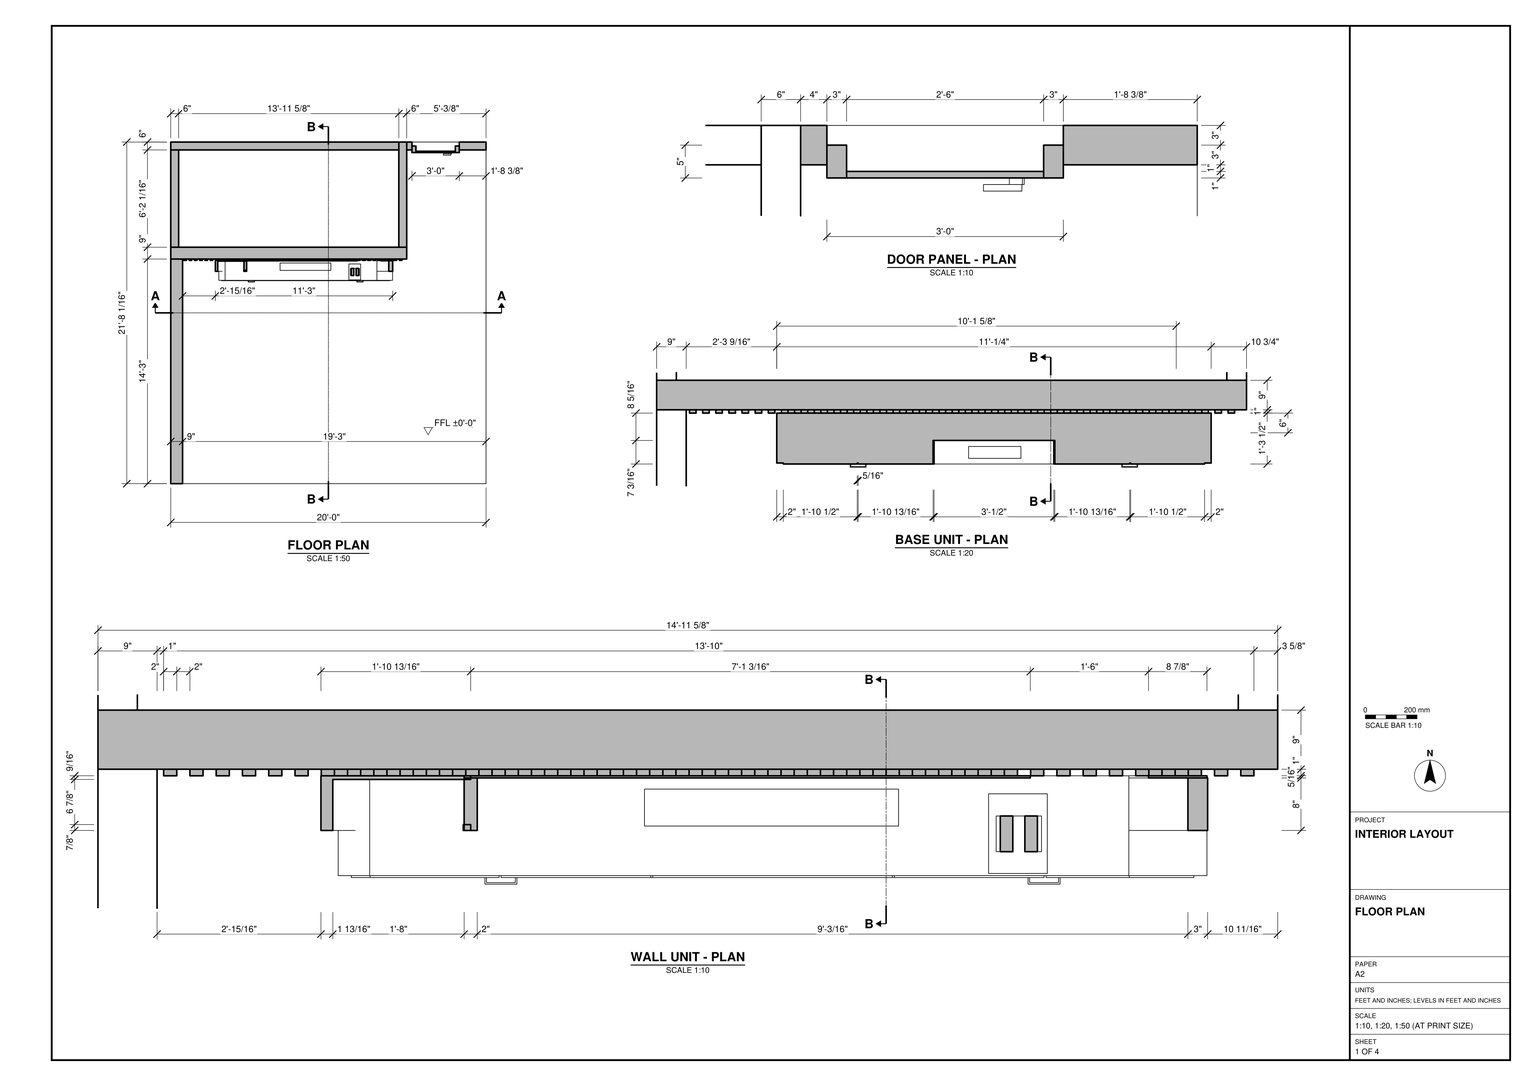
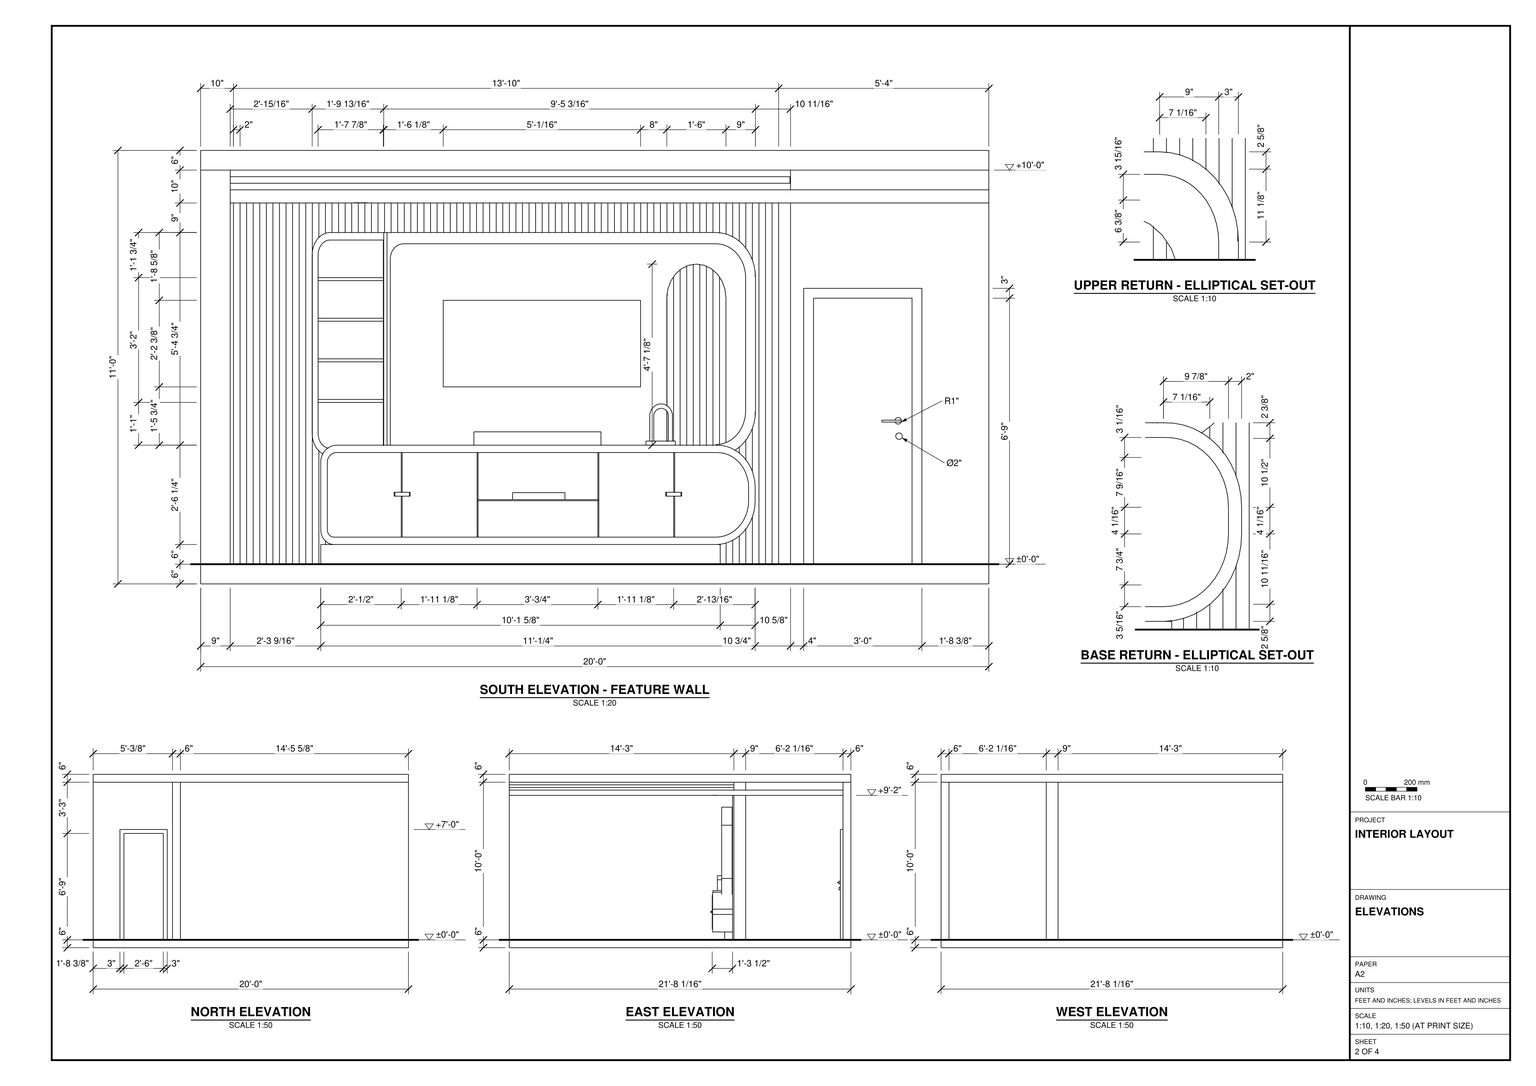
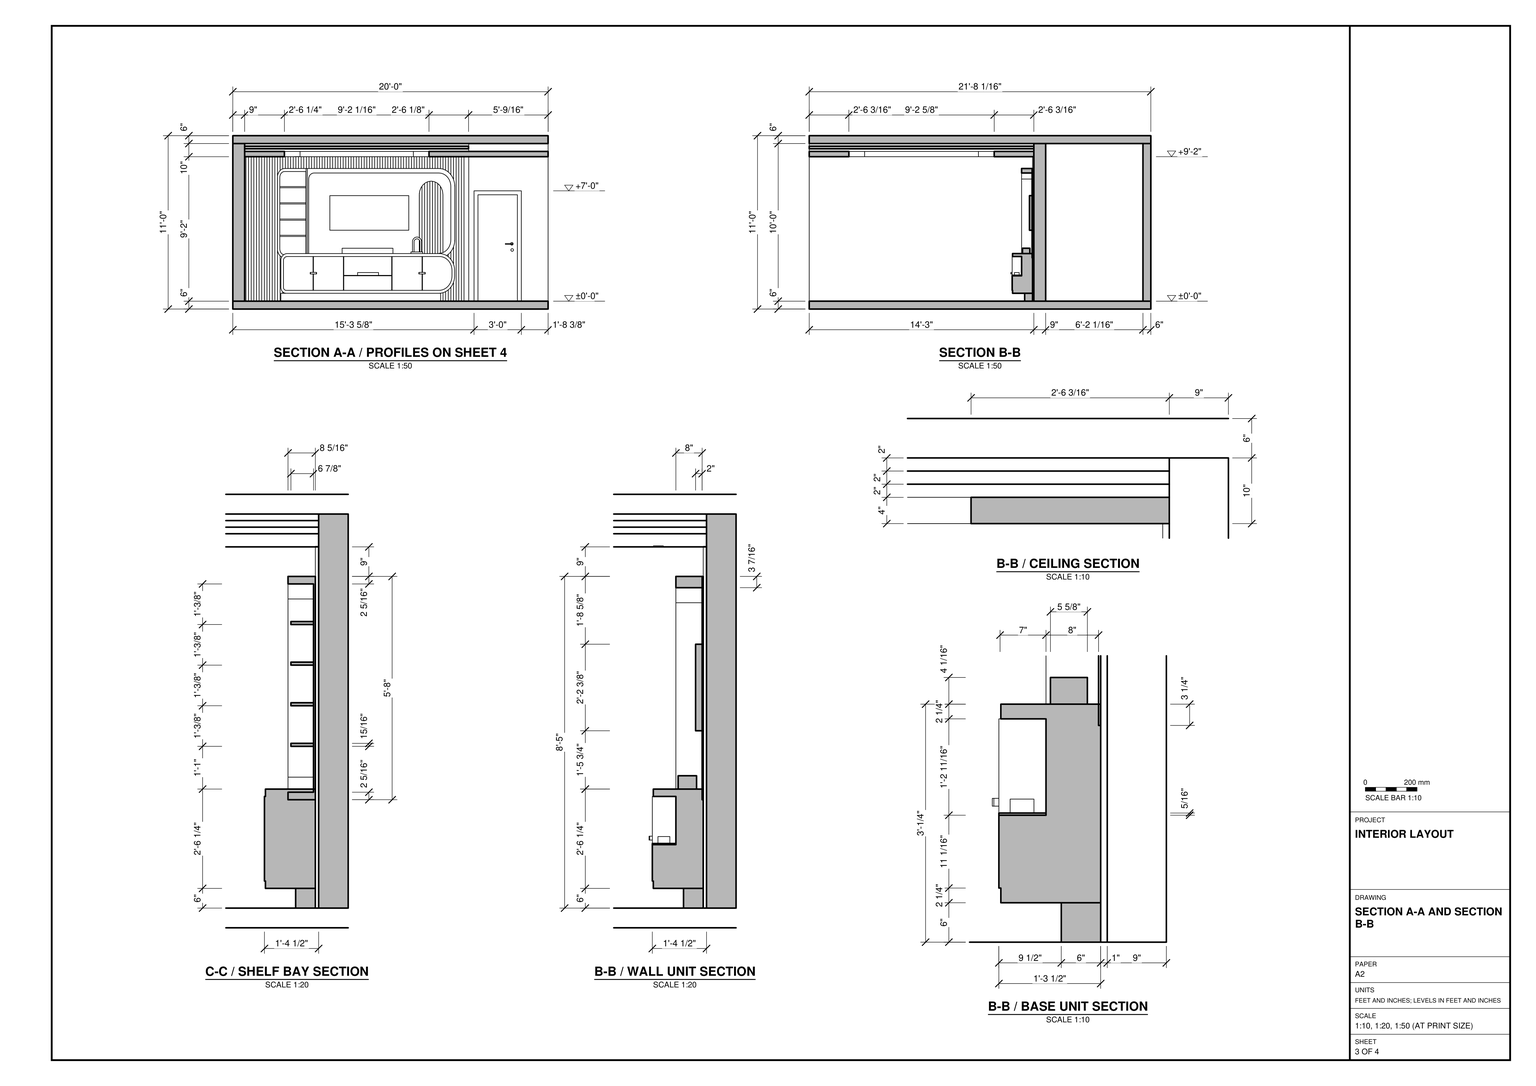
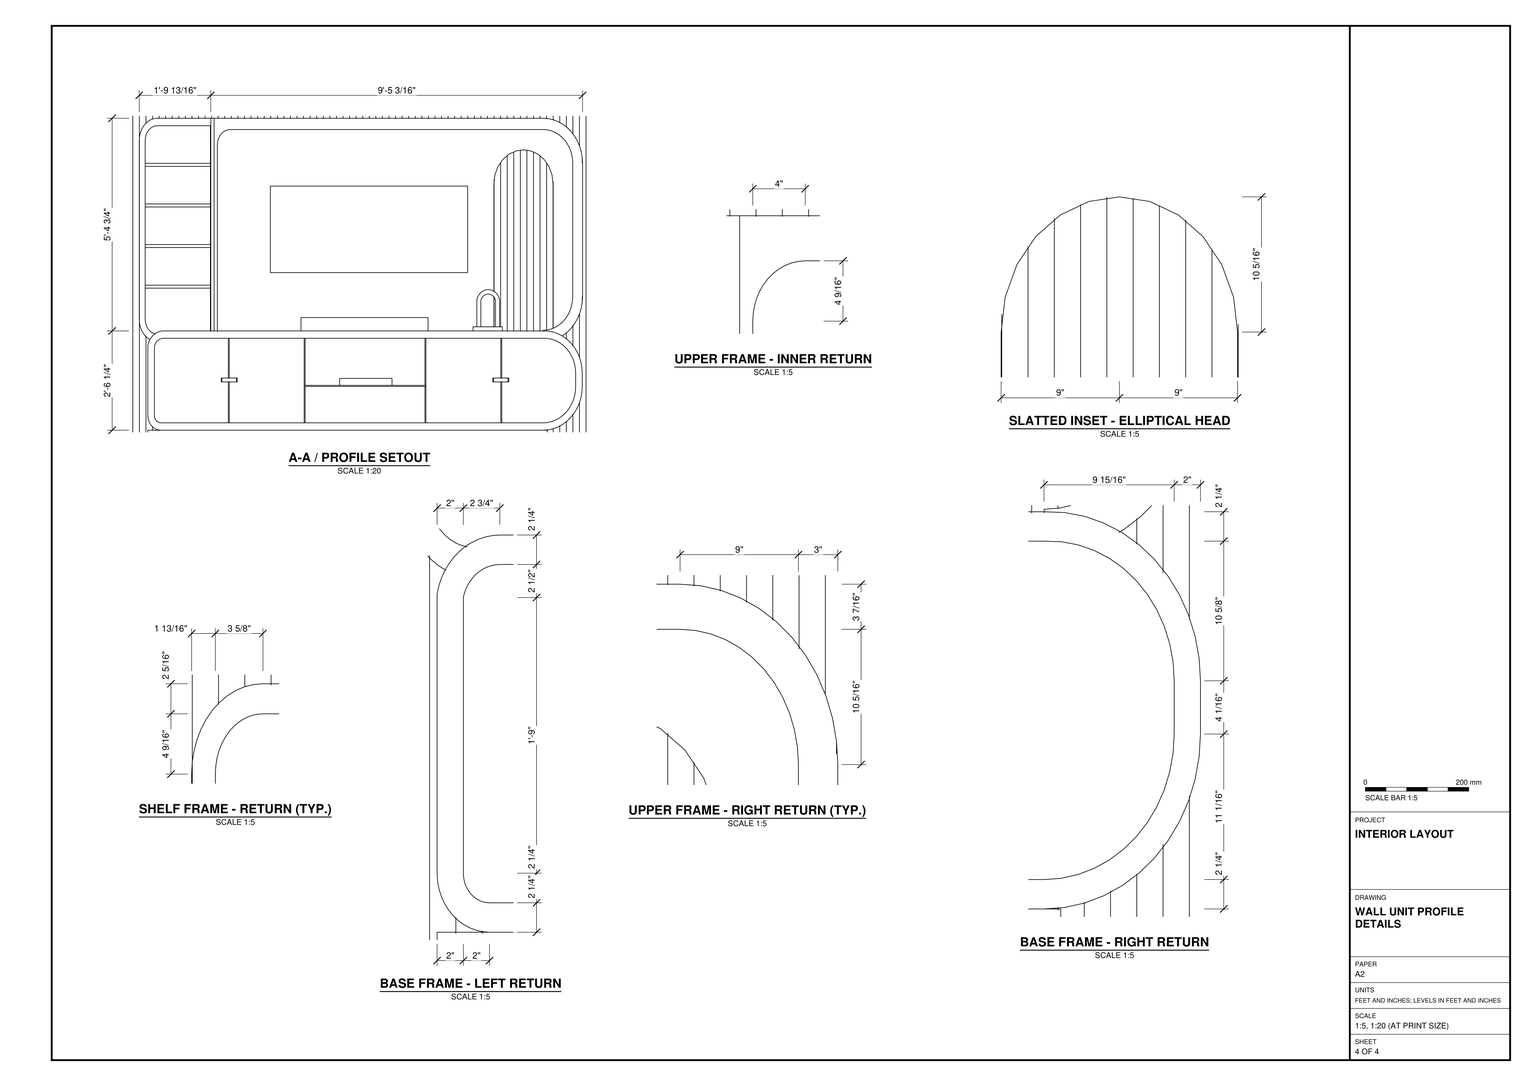
Build the single-storey interior in SketchUp using task_files/diagram_01.pdf. Work in feet and inches. The overall model is 20'-0" wide, 21'-8 1/16" deep and 11'-0" high, with the finished floor at ±0'-0".

Lay out the front room and the shallower space behind the transverse feature wall. Follow the plan for the 9" and 6" wall thicknesses, wall returns and framed door to the right of the joinery. Model the floor and upper slabs and the stepped ceiling below the upper slab, using the sections to set their heights.

Use the south elevation to lay out the vertical slats, low cabinet and upper wall unit. Set the cabinet on its recessed support and model its divided fronts, central recess and rounded right end. Above it, form the narrow open shelf bay on the left, the screen panel in the middle and the arched slatted inset on the right. Use the enlarged plans and sections for the joinery depths and the elliptical details for the curved returns. Decor and loose items may be any suitable library components.

Keep walls, slabs, ceiling and individual furniture or joinery pieces in separate groups or components, and use components for repeated parts. Save one SketchUp model as output_files/interior_with_a_curved_media_wall_and_fitted_cabinetry.skp.

# SketchUp Ruby script. Lengths in inches.
U = 1.inch
M = Sketchup.active_model
def pt(a) = Geom::Point3d.new(a.map { |v| v * U })
def face(e, loops, mat)
  f = e.add_face(loops[0].map { |a| pt(a) })
  loops[1..].each { |l| e.add_face(l.map { |a| pt(a) }).erase! }
  f.material = f.back_material = mat if mat
  f
end
# faces: each face lists its corners as indices into pts; further lists are holes
def faces(e, pts, list, mat = nil) = list.each { |f| face(e, (f[0].is_a?(Array) ? f : [f]).map { |l| l.map { |i| pts[i] } }, mat) }
# xy, xz, yz: faces in a plane at the given z, y or x. An outline is a flat list of corners, or four numbers for a rectangle; further outlines are holes
def ring(l) = l.size == 4 ? [[l[0], l[1]], [l[2], l[1]], [l[2], l[3]], [l[0], l[3]]] : l.each_slice(2).to_a
def flat(e, list, mat, &to3) = list.each { |f| face(e, (f[0].is_a?(Array) ? f : [f]).map { |l| ring(l).map { |u, v| to3.(u, v) } }, mat) }
def xy(e, z, list, mat = nil) = flat(e, list, mat) { |x, y| [x, y, z] }
def xz(e, y, list, mat = nil) = flat(e, list, mat) { |x, z| [x, y, z] }
def yz(e, x, list, mat = nil) = flat(e, list, mat) { |y, z| [x, y, z] }
def lines(e, pts, list) = list.each { |a, b| e.add_line(pt(pts[a]), pt(pts[b])) }
# prism: a flat outline (further loops are holes) pulled along v
def prism(e, loops, v, mat = nil)
  f = face(e, loops, mat); d = Geom::Vector3d.new(v.map { |x| x * U })
  f.pushpull(f.normal.samedirection?(d) ? d.length : -d.length)
end
def box(e, o, s, mat = nil) = prism(e, [[o, [o[0] + s[0], o[1], o[2]], [o[0] + s[0], o[1] + s[1], o[2]], [o[0], o[1] + s[1], o[2]]]], [0, 0, s[2]], mat)
def at(x, y, z, deg = 0) = Geom::Transformation.translation(pt([x, y, z])) * Geom::Transformation.rotation(ORIGIN, Z_AXIS, deg.degrees)
def axes(o, x, y, z) = Geom::Transformation.new([*x, 0, *y, 0, *z, 0, *pt(o).to_a, 1])
def part(name) = M.definitions.add(name)
# library, detail: a bought-in or finely detailed component or shape, given as its bounding box
def library(name, o, s) = part(name).tap { |d| box(d.entities, o, s) }
def detail(e, o, s) = box(e.add_group.entities, o, s)
def put(e, d, t, mat = nil) = e.add_instance(d, t).tap { |i| i.material = mat if mat }
def group(e, t, mat = nil) = e.add_group.tap { |g| g.transformation = t; g.material = mat if mat }.entities
root = M.entities
M.materials.add("[0118_Thistle]").color = [255, 225, 255]
M.materials.add("[0119_RosyBrown]").color = [96, 73, 73]
M.materials.add("[Color A01]").color = [255, 204, 204]
M.materials.add("[Color M08]").color = [30, 30, 30]
M.materials.add("[Color M09]").color = [0, 0, 0]
M.materials.add("[Wood Veneer 01]").color = [120, 70, 37]
c1 = library("Group\#11",[0,-15,0],[132.27,15.5,27])
c2 = part("Group\#15")
prism(c2.entities,[[[4.64,1,0],[4.875,1,0],[4.875,0,0],[0,0,0],[0,1,0],[0.23,1,0],[0.23,0.23,0],[4.64,0.23,0]]],[0,0,1.1875])
c3 = library("Group\#19",[0,0,0],[231,254.0625,4])
c4 = part("Group\#4")
box(c4.entities,[0,0,0],[2,1,108])
p = [[41.37,169.44,42],[55.74,169.44,42],[55.75,161.68,42],[56.75,161.68,42],[57.75,161.68,42],[57.75,169.5,42],
  [57.75,169.68,42],[141.95,169.5,42],[141.95,170,42.24],[141.95,169.68,42.24],[57.75,169.68,42.24],[57.75,161.68,42.24],
  [56.75,161.68,42.24],[55.75,161.68,42.24],[55.62,161.68,42.24],[55.62,162.57,42.24],[55.75,162.57,42.24],[55.75,169.44,42.24],
  [41.42,169.44,42.24],[41.37,170,42.24],[41.15,169.87,42.17],[40.92,169.76,42.1],[40.68,169.66,42.02],[40.44,169.58,41.95],
  [40.2,169.51,41.87],[39.95,169.45,41.79],[39.7,169.41,41.71],[39.44,169.39,41.63],[39.19,169.38,41.55],[38.9375,169.38,41.47],
  [38.68,169.41,41.39],[38.43,169.44,41.31],[38.43,161.68,41.31],[38.43,170,41.31]]
lines(root,p,[[0,1],[2,1],[2,3],[3,4],[4,5],[5,6],[5,7],[8,9],[9,10],[10,11],[11,12],[12,13],
  [13,14],[14,15],[15,16],[16,17],[17,18],[19,20],[20,21],[21,22],[22,23],[23,24],[24,25],[25,26],
  [26,27],[27,28],[28,29],[29,30],[30,31],[32,31],[31,33]])
g1 = group(root,at(0,-60,0))
box(g1,[0,60,0],[240,260.0625,6])
g2 = group(root,at(0,171,6),"[0119_RosyBrown]")
box(g2,[0,0,0],[179.62,9,120])
g3 = group(root,at(0,-60,6))
box(g3,[0,60,0],[9,171,120])
g4 = group(root,at(36.57,164,6),"[0118_Thistle]")
box(g4,[0,0,0],[121.64,6,6])
put(root,c1,axes([36.57,169.5,12],[1,0,0],[0,1,0],[0,0,1.12]),"[Color A01]")
g5 = group(root,at(33.95,161.67,39),"[Color A01]")
g6 = group(g5,at(1.81,0.89,16.26))
box(g6,[0,0,0],[19.86,6.875,0.92])
box(g6,[0,0,12.36],[19.86,6.875,0.92])
box(g6,[0,0,37.09],[19.86,6.875,0.92])
box(g6,[0,0,24.73],[19.86,6.875,0.91])
g7 = group(g5,at(0,8.03,0),"[Color A01]")
xy(g7,0,[[5.42,-8.03,22.8,0.29]],"[Color A01]")
xy(g7,2.29,[[5.42,-8.03,21.67,-8.03,21.67,-7.14,22.8,-7.14,22.8,-0.27,5.42,-0.27]],"[Color A01]")
xy(g7,65.71,[[5.42,-8.03,5.42,-0.27,22.8,-0.27,22.8,-7.14,21.67,-7.14,21.67,-8.03]],"[Color A01]")
xy(g7,68,[[5.42,-8.03,22.8,0.29]],"[Color A01]")
xz(g7,-8.03,[[5.42,0,5.42,2.29,4.95,2.33,4.48,2.45,4.04,2.64,3.61,2.9,3.22,3.24,2.86,3.63,2.55,4.08,2.29,4.58,2.08,5.12,1.93,5.68,1.84,6.27,1.81,6.87,1.81,61.13,1.84,61.73,1.93,62.32,2.08,62.88,2.29,63.42,2.55,63.92,2.86,64.37,3.22,64.77,3.61,65.1,4.04,65.36,4.48,65.56,4.95,65.67,5.42,65.71,21.67,65.71,21.67,2.29,5.42,2.29,5.42,0,22.8,0,22.8,68,5.42,68,4.71,67.94,4.02,67.77,3.34,67.48,2.71,67.08,2.12,66.58,1.59,65.99,1.12,65.3125,0.73,64.57,0.41,63.76,0.18,62.91,0.05,62.03,0,61.13,0,6.87,0.05,5.97,0.18,5.09,0.41,4.24,0.73,3.43,1.12,2.6875,1.59,2.01,2.12,1.42,2.71,0.92,3.34,0.52,4.02,0.23,4.71,0.06]],"[Color A01]")
xz(g7,-7.14,[[21.67,2.29,22.8,65.71]],"[Color A01]")
xz(g7,-0.27,[[5.42,2.29,22.8,2.29,22.8,65.71,5.42,65.71,4.95,65.67,4.48,65.56,4.04,65.36,3.61,65.1,3.22,64.77,2.86,64.37,2.55,63.92,2.29,63.42,2.08,62.88,1.93,62.32,1.84,61.73,1.81,61.13,1.81,6.87,1.84,6.27,1.93,5.68,2.08,5.12,2.29,4.58,2.55,4.08,2.86,3.63,3.22,3.24,3.61,2.9,4.04,2.64,4.48,2.45,4.95,2.33]],"[Color A01]")
xz(g7,0.29,[[5.42,0,4.71,0.06,4.02,0.23,3.34,0.52,2.71,0.92,2.12,1.42,1.59,2.01,1.12,2.6875,0.73,3.43,0.41,4.24,0.18,5.09,0.05,5.97,0,6.87,0,61.13,0.05,62.03,0.18,62.91,0.41,63.76,0.73,64.57,1.12,65.3125,1.59,65.99,2.12,66.58,2.71,67.08,3.34,67.48,4.02,67.77,4.71,67.94,5.42,68,22.8,68,22.8,0]],"[Color A01]")
yz(g7,0,[[-8.03,6.87,0.29,61.13]],"[Color A01]")
yz(g7,1.81,[[-8.03,6.87,-0.27,61.13]],"[Color A01]")
yz(g7,21.67,[[-8.03,2.29,-7.14,65.71]],"[Color A01]")
yz(g7,22.8,[[[-8.03,0,0.29,68],[-7.14,2.29,-0.27,65.71]]],"[Color A01]")
# 1 loose lines left out
p = [[4.71,0.29,0.06],[5.42,0.29,0],[5.42,-8.03,0],[4.71,-8.03,0.06],[4.02,0.29,0.23],[4.02,-8.03,0.23],
  [3.34,0.29,0.52],[3.34,-8.03,0.52],[2.71,0.29,0.92],[2.71,-8.03,0.92],[2.12,0.29,1.42],[2.12,-8.03,1.42],
  [1.59,0.29,2.01],[1.59,-8.03,2.01],[1.12,0.29,2.6875],[1.12,-8.03,2.6875],[4.95,-0.27,2.33],[4.48,-0.27,2.45],
  [4.48,-8.03,2.45],[4.95,-8.03,2.33],[5.42,-0.27,2.29],[5.42,-8.03,2.29],[4.04,-0.27,2.64],[4.04,-8.03,2.64],
  [3.61,-0.27,2.9],[3.61,-8.03,2.9],[0.73,0.29,3.43],[0.73,-8.03,3.43],[3.22,-0.27,3.24],[3.22,-8.03,3.24],
  [2.86,-0.27,3.63],[2.86,-8.03,3.63],[0.41,0.29,4.24],[0.41,-8.03,4.24],[2.55,-0.27,4.08],[2.55,-8.03,4.08],
  [2.29,-0.27,4.58],[2.29,-8.03,4.58],[0.18,0.29,5.09],[0.18,-8.03,5.09],[2.08,-0.27,5.12],[2.08,-8.03,5.12],
  [0.05,0.29,5.97],[0.05,-8.03,5.97],[1.93,-0.27,5.68],[1.93,-8.03,5.68],[1.84,-0.27,6.27],[1.84,-8.03,6.27],
  [0,0.29,6.87],[0,-8.03,6.87],[1.81,-0.27,6.87],[1.81,-8.03,6.87],[0.05,0.29,62.03],[0,0.29,61.13],
  [0,-8.03,61.13],[0.05,-8.03,62.03],[1.81,-0.27,61.13],[1.84,-0.27,61.73],[1.84,-8.03,61.73],[1.81,-8.03,61.13],
  [1.93,-0.27,62.32],[1.93,-8.03,62.32],[0.18,0.29,62.91],[0.18,-8.03,62.91],[2.08,-0.27,62.88],[2.08,-8.03,62.88],
  [0.41,0.29,63.76],[0.41,-8.03,63.76],[2.29,-0.27,63.42],[2.29,-8.03,63.42],[2.55,-0.27,63.92],[2.55,-8.03,63.92],
  [0.73,0.29,64.57],[0.73,-8.03,64.57],[2.86,-0.27,64.37],[2.86,-8.03,64.37],[3.22,-0.27,64.77],[3.22,-8.03,64.77],
  [1.12,0.29,65.3125],[1.12,-8.03,65.3125],[3.61,-0.27,65.1],[3.61,-8.03,65.1],[4.04,-0.27,65.36],[4.04,-8.03,65.36],
  [1.59,0.29,65.99],[1.59,-8.03,65.99],[4.48,-0.27,65.56],[4.48,-8.03,65.56],[4.95,-0.27,65.67],[4.95,-8.03,65.67],
  [5.42,-0.27,65.71],[5.42,-8.03,65.71],[2.12,0.29,66.58],[2.12,-8.03,66.58],[2.71,0.29,67.08],[2.71,-8.03,67.08],
  [3.34,0.29,67.48],[3.34,-8.03,67.48],[4.02,0.29,67.77],[4.02,-8.03,67.77],[4.71,0.29,67.94],[4.71,-8.03,67.94],
  [5.42,0.29,68],[5.42,-8.03,68]]
faces(g7,p,[[0,1,2,3],[4,0,3,5],[6,4,5,7],[8,6,7,9],[10,8,9,11],[12,10,11,13],[14,12,13,15],[16,17,18,19],
  [20,16,19,21],[17,22,23,18],[22,24,25,23],[26,14,15,27],[24,28,29,25],[28,30,31,29],[32,26,27,33],[30,34,35,31],
  [34,36,37,35],[38,32,33,39],[36,40,41,37],[42,38,39,43],[40,44,45,41],[44,46,47,45],[48,42,43,49],[46,50,51,47],
  [52,53,54,55],[56,57,58,59],[57,60,61,58],[62,52,55,63],[60,64,65,61],[66,62,63,67],[64,68,69,65],[68,70,71,69],
  [72,66,67,73],[70,74,75,71],[74,76,77,75],[78,72,73,79],[76,80,81,77],[80,82,83,81],[84,78,79,85],[82,86,87,83],
  [86,88,89,87],[88,90,91,89],[92,84,85,93],[94,92,93,95],[96,94,95,97],[98,96,97,99],[100,98,99,101],[102,100,101,103]],"[Color A01]")
put(root,c2,at(58.91,153.5,26.71),"[Color M09]")
put(root,c2,at(141.61,153.5,26.71),"[Color M09]")
g8 = group(root,at(83.21,162.35,42.24),"[Color M09]")
box(g8,[0,0,0],[38.6875,5.625,4.0625])
g9 = group(root,at(94.98,156.22,25.66),"[Color M09]")
box(g9,[0,0,0],[15.9375,3.625,2.125])
g10 = group(root,at(73.87,167.68,60),"[Color M08]")
box(g10,[0,0,0],[60.08,2,26.35])
g11 = group(root,at(9,0,122),"[0118_Thistle]")
box(g11,[0,0,0],[170.45,171,2])
put(root,c3,at(9,0,116),"[0118_Thistle]")
g12 = group(root,at(10,170,6),"[0119_RosyBrown]")
put(g12,c4,axes([160,0,0],[1,0,0],[0,1,0],[0,0,1.02]))
put(g12,c4,axes([136,0,0],[1,0,0],[0,1,0],[0,0,1.02]))
put(g12,c4,axes([156,0,0],[1,0,0],[0,1,0],[0,0,1.02]))
put(g12,c4,axes([164,0,0],[1,0,0],[0,1,0],[0,0,1.02]))
put(g12,c4,axes([132,0,0],[1,0,0],[0,1,0],[0,0,1.02]))
put(g12,c4,axes([148,0,0],[1,0,0],[0,1,0],[0,0,1.02]))
put(g12,c4,axes([140,0,0],[1,0,0],[0,1,0],[0,0,1.02]))
put(g12,c4,axes([144,0,0],[1,0,0],[0,1,0],[0,0,1.02]))
put(g12,c4,axes([152,0,0],[1,0,0],[0,1,0],[0,0,1.02]))
put(g12,c4,axes([24,0,0],[1,0,0],[0,1,0],[0,0,1.02]))
put(g12,c4,axes([76,0,0],[1,0,0],[0,1,0],[0,0,1.02]))
put(g12,c4,axes([60,0,0],[1,0,0],[0,1,0],[0,0,1.02]))
put(g12,c4,axes([52,0,0],[1,0,0],[0,1,0],[0,0,1.02]))
put(g12,c4,axes([12,0,0],[1,0,0],[0,1,0],[0,0,1.02]))
put(g12,c4,axes([112,0,0],[1,0,0],[0,1,0],[0,0,1.02]))
put(g12,c4,axes([16,0,0],[1,0,0],[0,1,0],[0,0,1.02]))
put(g12,c4,axes([36,0,0],[1,0,0],[0,1,0],[0,0,1.02]))
put(g12,c4,axes([72,0,0],[1,0,0],[0,1,0],[0,0,1.02]))
put(g12,c4,axes([20,0,0],[1,0,0],[0,1,0],[0,0,1.02]))
put(g12,c4,axes([44,0,0],[1,0,0],[0,1,0],[0,0,1.02]))
put(g12,c4,axes([64,0,0],[1,0,0],[0,1,0],[0,0,1.02]))
put(g12,c4,axes([56,0,0],[1,0,0],[0,1,0],[0,0,1.02]))
put(g12,c4,axes([4,0,0],[1,0,0],[0,1,0],[0,0,1.02]))
put(g12,c4,axes([80,0,0],[1,0,0],[0,1,0],[0,0,1.02]))
put(g12,c4,axes([68,0,0],[1,0,0],[0,1,0],[0,0,1.02]))
put(g12,c4,axes([8,0,0],[1,0,0],[0,1,0],[0,0,1.02]))
put(g12,c4,axes([32,0,0],[1,0,0],[0,1,0],[0,0,1.02]))
put(g12,c4,axes([48,0,0],[1,0,0],[0,1,0],[0,0,1.02]))
put(g12,c4,axes([40,0,0],[1,0,0],[0,1,0],[0,0,1.02]))
put(g12,c4,axes([28,0,0],[1,0,0],[0,1,0],[0,0,1.02]))
put(g12,c4,axes([92,0,0],[1,0,0],[0,1,0],[0,0,1.02]))
put(g12,c4,axes([84,0,0],[1,0,0],[0,1,0],[0,0,1.02]))
put(g12,c4,axes([0,0,0],[1,0,0],[0,1,0],[0,0,1.02]))
put(g12,c4,axes([88,0,0],[1,0,0],[0,1,0],[0,0,1.02]))
put(g12,c4,axes([124,0,0],[1,0,0],[0,1,0],[0,0,1.02]))
put(g12,c4,axes([128,0,0],[1,0,0],[0,1,0],[0,0,1.02]))
put(g12,c4,axes([96,0,0],[1,0,0],[0,1,0],[0,0,1.02]))
put(g12,c4,axes([108,0,0],[1,0,0],[0,1,0],[0,0,1.02]))
put(g12,c4,axes([104,0,0],[1,0,0],[0,1,0],[0,0,1.02]))
put(g12,c4,axes([120,0,0],[1,0,0],[0,1,0],[0,0,1.02]))
put(g12,c4,axes([100,0,0],[1,0,0],[0,1,0],[0,0,1.02]))
put(g12,c4,axes([116,0,0],[1,0,0],[0,1,0],[0,0,1.02]))
g13 = group(root,at(173.62,180,6),"[Color A01]")
box(g13,[0,0,0],[6,80.0625,120])
g14 = group(root,at(179.62,254.0625,6),"[Color A01]")
prism(g14,[[[60.38,6,0],[40,6,0],[40,6,84],[4,6,84],[4,6,0],[0,6,0],[0,6,120],[60.38,6,120]]],[0,-6,0])
g15 = group(root,at(183.62,254.0625,6),"[Wood Veneer 01]")
g16 = group(g15,at(0,0,0))
prism(g16,[[[36,3,0],[33,3,0],[33,3,81],[3,3,81],[3,3,0],[0,3,0],[0,3,84],[36,3,84]]],[0,-5,0])
g17 = group(g15,at(3,-2,0))
box(g17,[0,0,0],[30,1,81])
g18 = group(root,at(211.65,251.0625,43.99))
prism(g18,[[[1,1,0],[0.74,1,0.03],[0.5,1,0.13],[0.29,1,0.29],[0.13,1,0.5],[0.03,1,0.74],[0,1,1],[0.03,1,1.26],[0.13,1,1.5],[0.29,1,1.71],[0.5,1,1.87],[0.74,1,1.97],[1,1,2],[1.26,1,1.97],[1.5,1,1.87],[1.71,1,1.71],[1.87,1,1.5],[1.97,1,1.26],[2,1,1],[1.97,1,0.74],[1.87,1,0.5],[1.71,1,0.29],[1.5,1,0.13],[1.26,1,0.03]]],[0,-1,0])
g19 = group(root,at(207.46,250.0625,48.67))
g20 = group(g19,at(3.9375,1,0))
prism(g20,[[[1.6,1,0.2],[1.375,1,0.07],[1.12,1,0],[0.86,1,0],[0.61,1,0.07],[0.38,1,0.2],[0.2,1,0.38],[0.07,1,0.61],[0,1,0.86],[0,1,1.12],[0.07,1,1.375],[0.2,1,1.6],[0.38,1,1.78],[0.61,1,1.92],[0.86,1,1.98],[1.12,1,1.98],[1.375,1,1.92],[1.6,1,1.78],[1.78,1,1.6],[1.92,1,1.375],[1.98,1,1.12],[1.98,1,0.86],[1.92,1,0.61],[1.78,1,0.38]]],[0,-1,0])
g21 = group(g19,at(0,0,0.61))
box(g21,[0,0,0],[5.85,1,0.58])
g22 = group(root,at(0,0,126))
box(g22,[0,0,0],[240,260.0625,6])
g23 = group(root,at(0,254.0625,6))
box(g23,[0,0,0],[173.62,6,120])
g24 = group(root,at(0,180,6))
box(g24,[0,0,0],[6,74.0625,120])
g25 = group(root,at(136.22,156.44,42.24),"[0119_RosyBrown]")
box(g25,[-0.625,-1.3125,0],[8.9375,12.125,1.25])
g26 = group(root,at(55.75,161.68,39),"[Color A01]")
g27 = group(g26,at(0,0,0))
prism(g27,[[[102.77,8,0.12],[101.2,8,0],[101.2,8,3.43],[102.375,8,3.52],[103.53,8,3.79],[104.64,8,4.22],[105.7,8,4.81],[106.68,8,5.5625],[107.5625,8,6.45],[108.34,8,7.47],[108.99,8,8.59],[109.51,8,9.79],[109.89,8,11.07],[110.125,8,12.39],[110.2,8,13.74],[110.2,8,54.26],[110.125,8,55.61],[109.89,8,56.93],[109.51,8,58.21],[108.99,8,59.42],[108.34,8,60.54],[107.5625,8,61.55],[106.68,8,62.4375],[105.7,8,63.1875],[104.64,8,63.78],[103.53,8,64.22],[102.375,8,64.48],[101.2,8,64.57],[6,8,64.57],[5.48,8,64.53],[4.96,8,64.41],[4.47,8,64.22],[4,8,63.95],[3.56,8,63.62],[3.17,8,63.23],[2.83,8,62.78],[2.54,8,62.28],[2.3,8,61.74],[2.14,8,61.17],[2.03,8,60.59],[2,8,59.99],[2,8,0],[0,8,0],[0,8,68],[101.2,8,68],[102.77,8,67.88],[104.31,8,67.53],[105.79,8,66.96],[107.2,8,66.16],[108.51,8,65.16],[109.69,8,63.98],[110.72,8,62.625],[111.59,8,61.13],[112.29,8,59.52],[112.79,8,57.82],[113.1,8,56.06],[113.2,8,54.26],[113.2,8,13.74],[113.1,8,11.94],[112.79,8,10.18],[112.29,8,8.48],[111.59,8,6.87],[110.72,8,5.375],[109.69,8,4.02],[108.51,8,2.84],[107.2,8,1.84],[105.79,8,1.05],[104.31,8,0.47]]],[0,-8,0])
g28 = group(g26,at(0,8,0))
xy(g28,0,[[0,0,86.2,0.32]])
xy(g28,68,[[0,0,101.2,0.32]])
xz(g28,0,[[0,0,86.2,0,86.2,48.08,86.51,50.75,87.41,53.23,88.84,55.37,90.7,57,92.87,58.03,95.2,58.38,97.53,58.03,99.7,57,101.5625,55.37,102.99,53.23,103.89,50.75,104.2,48.08,104.2,0.44,104.31,0.47,105.79,1.05,107.2,1.84,108.51,2.84,109.69,4.02,110.72,5.375,111.59,6.87,112.29,8.48,112.79,10.18,113.1,11.94,113.1,56.06,112.79,57.82,112.29,59.52,111.59,61.13,110.72,62.625,109.69,63.98,108.51,65.16,107.2,66.16,105.79,66.96,104.31,67.53,102.77,67.88,101.2,68,0,68],[101.2,0,104.2,0,104.2,0.44,102.77,0.12]])
xz(g28,0.32,[[0,0,0,68,101.2,68,102.77,67.88,104.31,67.53,105.79,66.96,107.2,66.16,108.51,65.16,109.69,63.98,110.72,62.625,111.59,61.13,112.29,59.52,112.79,57.82,113.1,56.06,113.1,11.94,112.79,10.18,112.29,8.48,111.59,6.87,110.72,5.375,109.69,4.02,108.51,2.84,107.2,1.84,105.79,1.05,104.31,0.47,104.2,0.44,104.2,48.08,103.89,50.75,102.99,53.23,101.5625,55.37,99.7,57,97.53,58.03,95.2,58.38,92.87,58.03,90.7,57,88.84,55.37,87.41,53.23,86.51,50.75,86.2,48.08,86.2,0]])
yz(g28,0,[[0,0,0.32,68]])
yz(g28,86.2,[[0,0,0.32,48.08]])
yz(g28,104.2,[[0,0.44,0.32,48.08]])
yz(g28,113.1,[[0,11.94,0.32,56.06]])
# 2 loose lines left out
p = [[101.2,0,0],[102.77,0,0.12],[102.77,0.32,0.12],[101.2,0.32,0],[104.2,0,0.44],[104.2,0.32,0.44],
  [104.31,0,0.47],[104.31,0.32,0.47],[105.79,0,1.05],[105.79,0.32,1.05],[107.2,0,1.84],[107.2,0.32,1.84],
  [108.51,0,2.84],[108.51,0.32,2.84],[109.69,0,4.02],[109.69,0.32,4.02],[110.72,0,5.375],[110.72,0.32,5.375],
  [111.59,0,6.87],[111.59,0.32,6.87],[112.29,0,8.48],[112.29,0.32,8.48],[112.79,0,10.18],[112.79,0.32,10.18],
  [113.1,0,11.94],[113.1,0.32,11.94],[86.51,0,50.75],[86.2,0,48.08],[86.2,0.32,48.08],[86.51,0.32,50.75],
  [104.2,0,48.08],[103.89,0,50.75],[103.89,0.32,50.75],[104.2,0.32,48.08],[87.41,0,53.23],[87.41,0.32,53.23],
  [102.99,0,53.23],[102.99,0.32,53.23],[88.84,0,55.37],[88.84,0.32,55.37],[101.5625,0,55.37],[101.5625,0.32,55.37],
  [90.7,0,57],[90.7,0.32,57],[99.7,0,57],[99.7,0.32,57],[112.79,0,57.82],[113.1,0,56.06],
  [113.1,0.32,56.06],[112.79,0.32,57.82],[92.87,0,58.03],[92.87,0.32,58.03],[97.53,0,58.03],[97.53,0.32,58.03],
  [112.29,0,59.52],[112.29,0.32,59.52],[95.2,0,58.38],[95.2,0.32,58.38],[111.59,0,61.13],[111.59,0.32,61.13],
  [110.72,0,62.625],[110.72,0.32,62.625],[109.69,0,63.98],[109.69,0.32,63.98],[108.51,0,65.16],[108.51,0.32,65.16],
  [107.2,0,66.16],[107.2,0.32,66.16],[105.79,0,66.96],[105.79,0.32,66.96],[104.31,0,67.53],[104.31,0.32,67.53],
  [102.77,0,67.88],[102.77,0.32,67.88],[101.2,0,68],[101.2,0.32,68]]
faces(g28,p,[[0,1,2,3],[4,1,2,5],[6,4,5,7],[8,6,7,9],[10,8,9,11],[12,10,11,13],[14,12,13,15],[16,14,15,17],
  [18,16,17,19],[20,18,19,21],[22,20,21,23],[24,22,23,25],[26,27,28,29],[30,31,32,33],[34,26,29,35],[31,36,37,32],
  [38,34,35,39],[36,40,41,37],[42,38,39,43],[40,44,45,41],[46,47,48,49],[50,42,43,51],[44,52,53,45],[54,46,49,55],
  [56,50,51,57],[52,56,57,53],[58,54,55,59],[60,58,59,61],[62,60,61,63],[64,62,63,65],[66,64,65,67],[68,66,67,69],
  [70,68,69,71],[72,70,71,73],[74,72,73,75]])
g29 = group(root,at(136.75,158.44,43.49),"[Color M09]")
prism(g29,[[[1.22,5.4375,0],[0,5.4375,0],[0,5.4375,8.25],[0.26,5.4375,9.09],[0.68,5.4375,9.85],[1.24,5.4375,10.48],[1.91,5.4375,10.95],[2.66,5.4375,11.25],[3.45,5.4375,11.35],[4.24,5.4375,11.25],[5,5.4375,10.95],[5.67,5.4375,10.48],[6.23,5.4375,9.85],[6.65,5.4375,9.09],[6.91,5.4375,8.25],[6.91,5.4375,0],[5.69,5.4375,0],[5.69,5.4375,8.02],[5.54,5.4375,8.5],[5.27,5.4375,9],[4.9,5.4375,9.41],[4.46,5.4375,9.72],[3.97,5.4375,9.91],[3.45,5.4375,9.98],[2.9375,5.4375,9.91],[2.45,5.4375,9.72],[2.01,5.4375,9.41],[1.64,5.4375,9],[1.36,5.4375,8.5],[1.22,5.4375,8.02]]],[0,-5.4375,0])
# 1 loose lines left out
